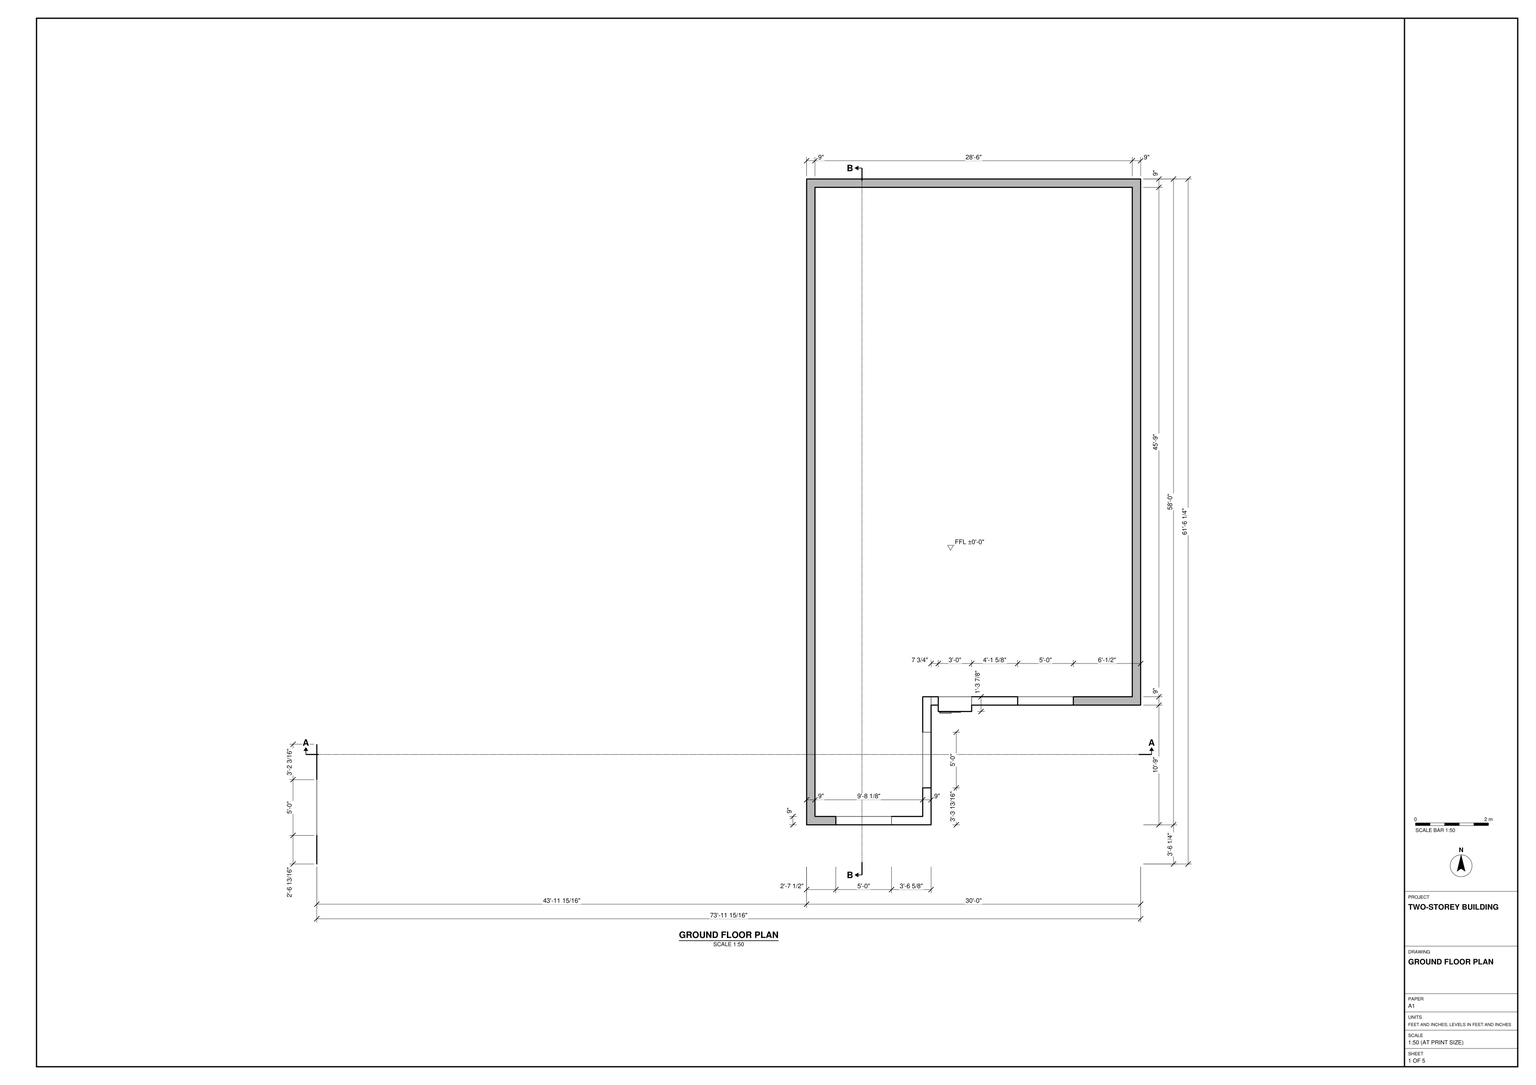
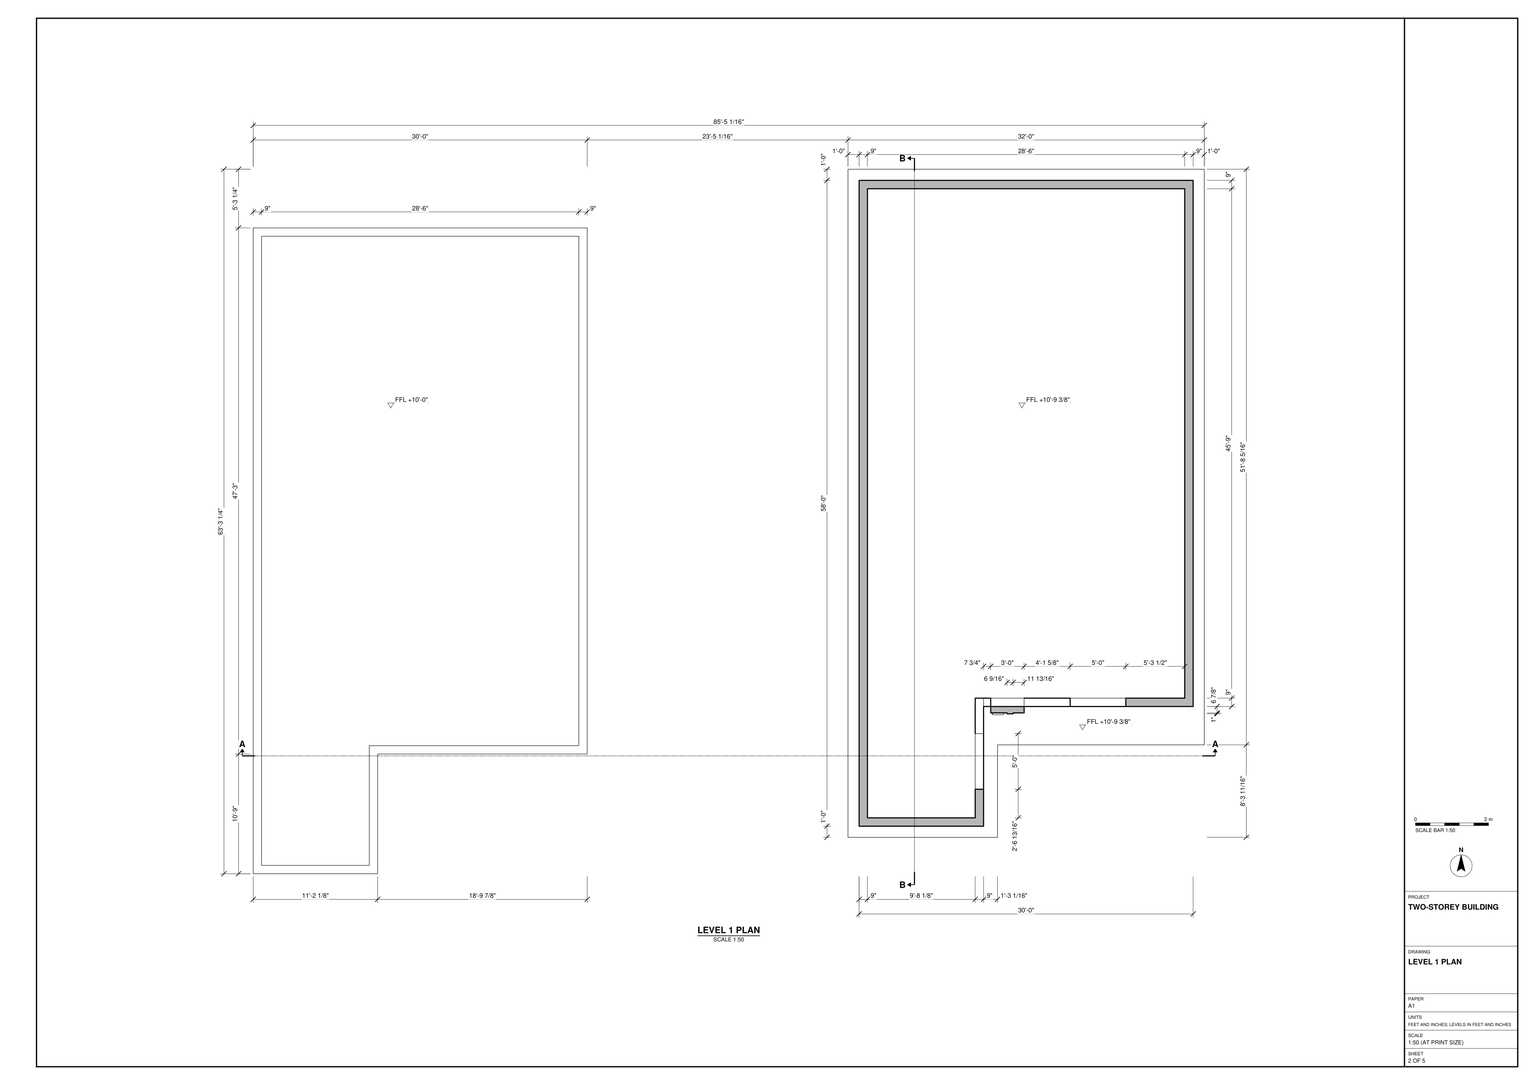
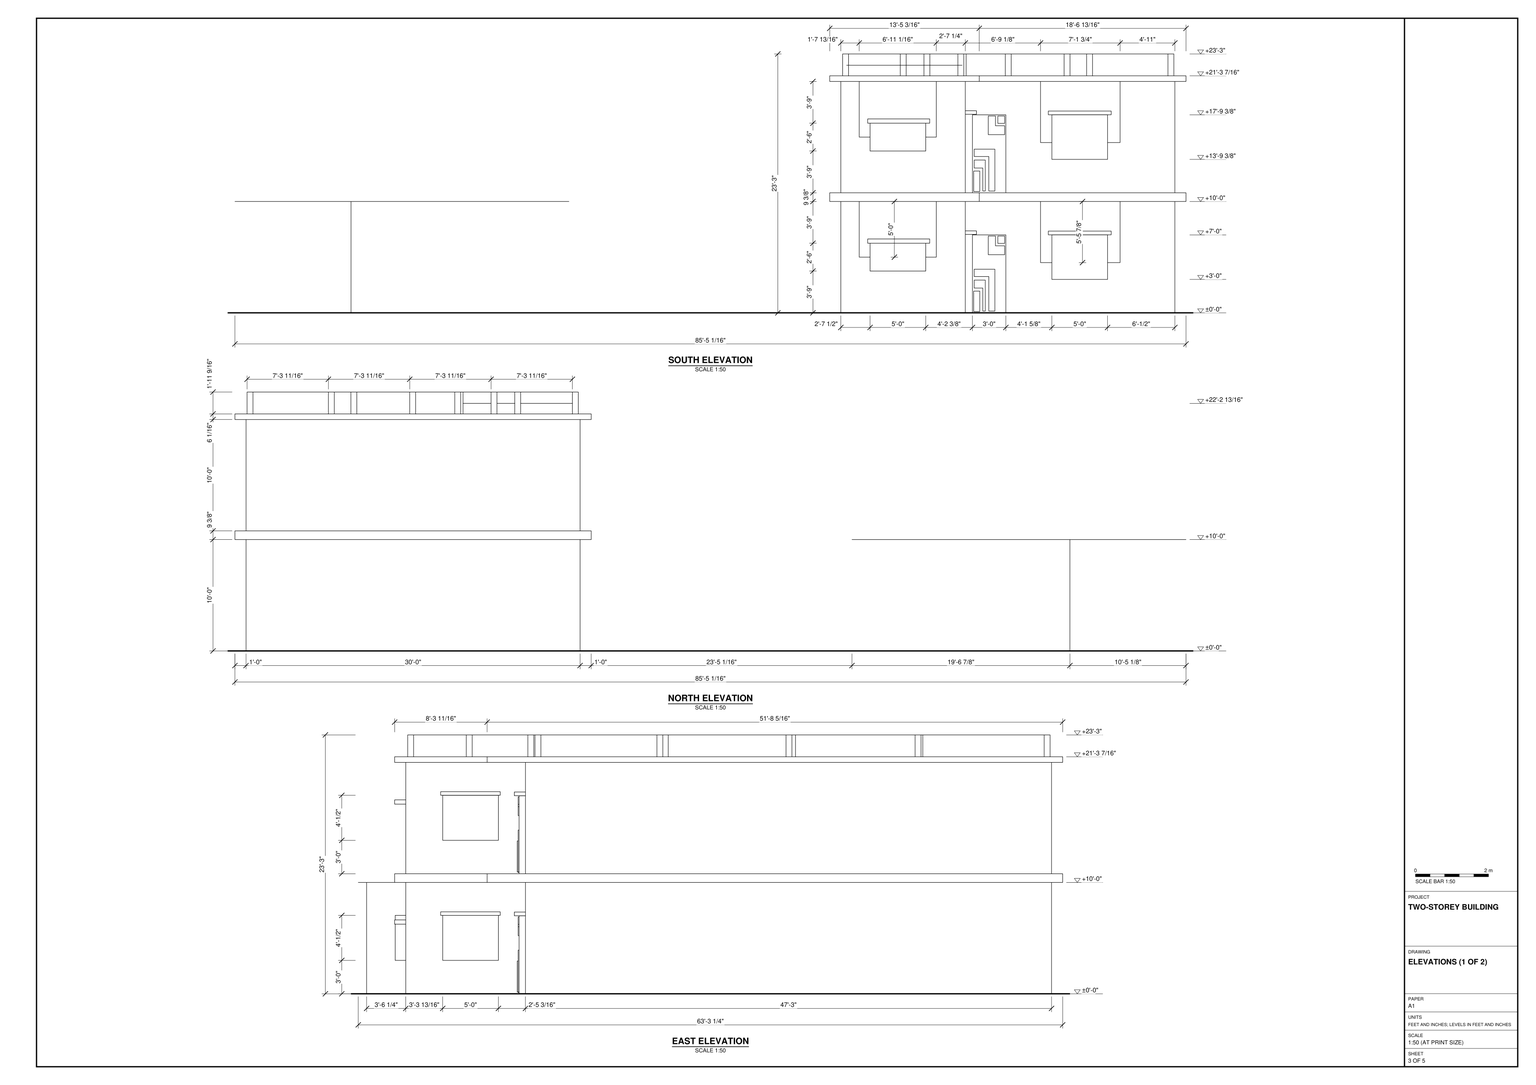
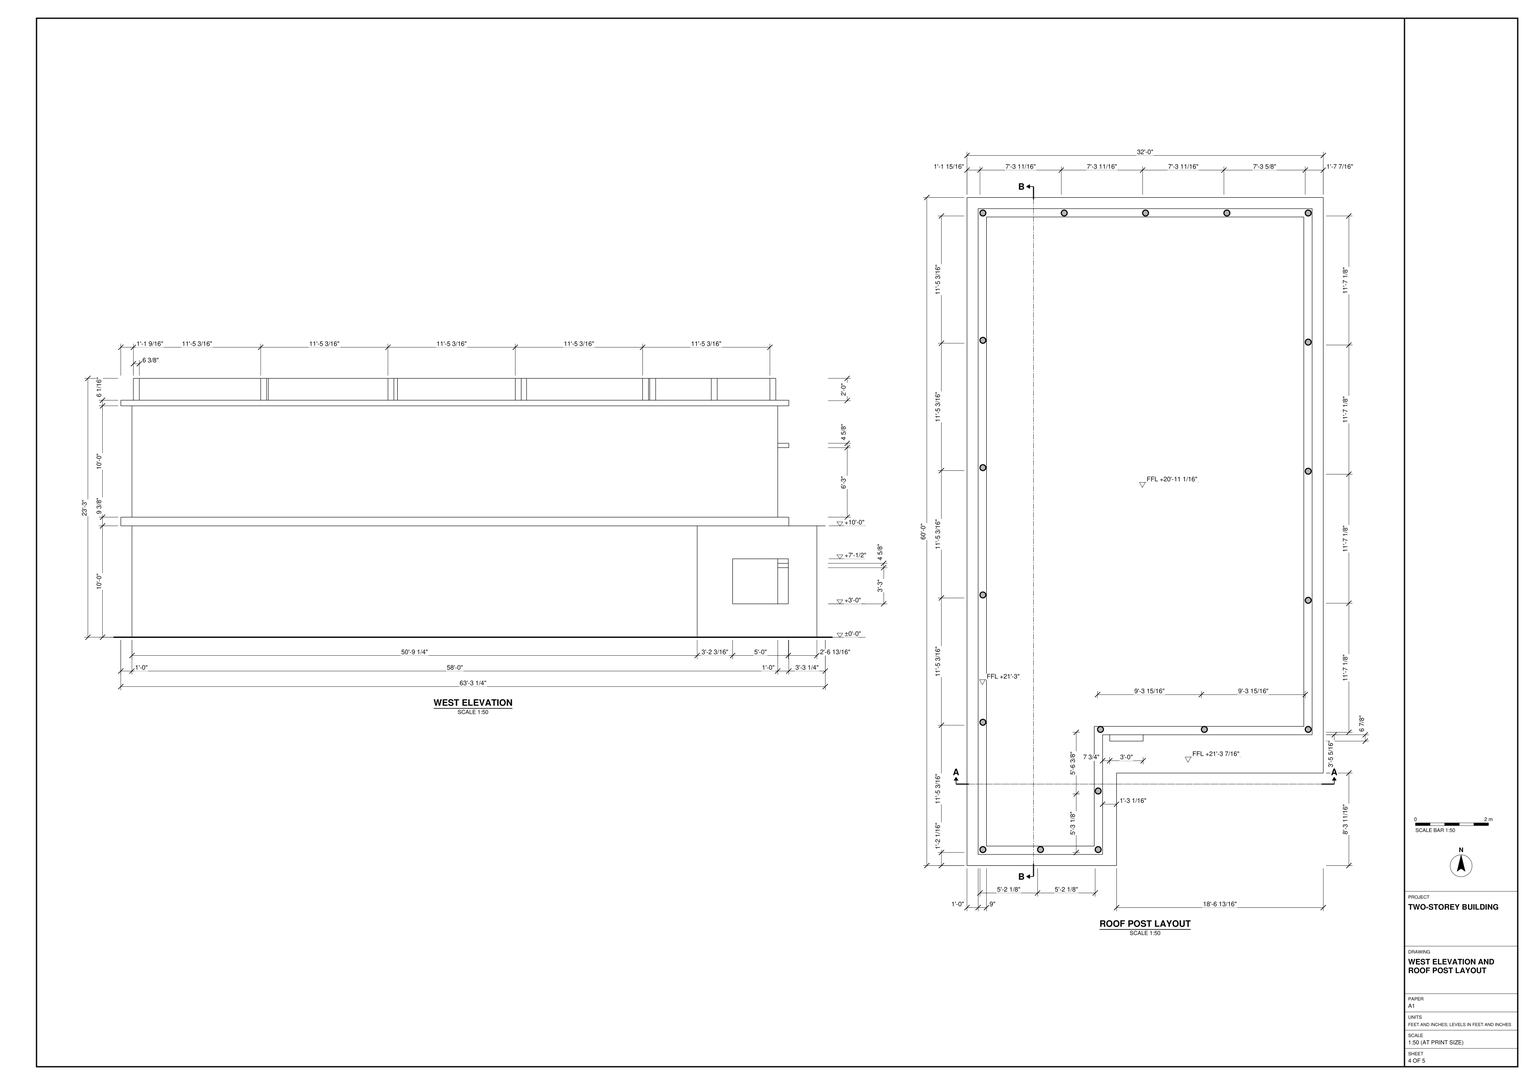
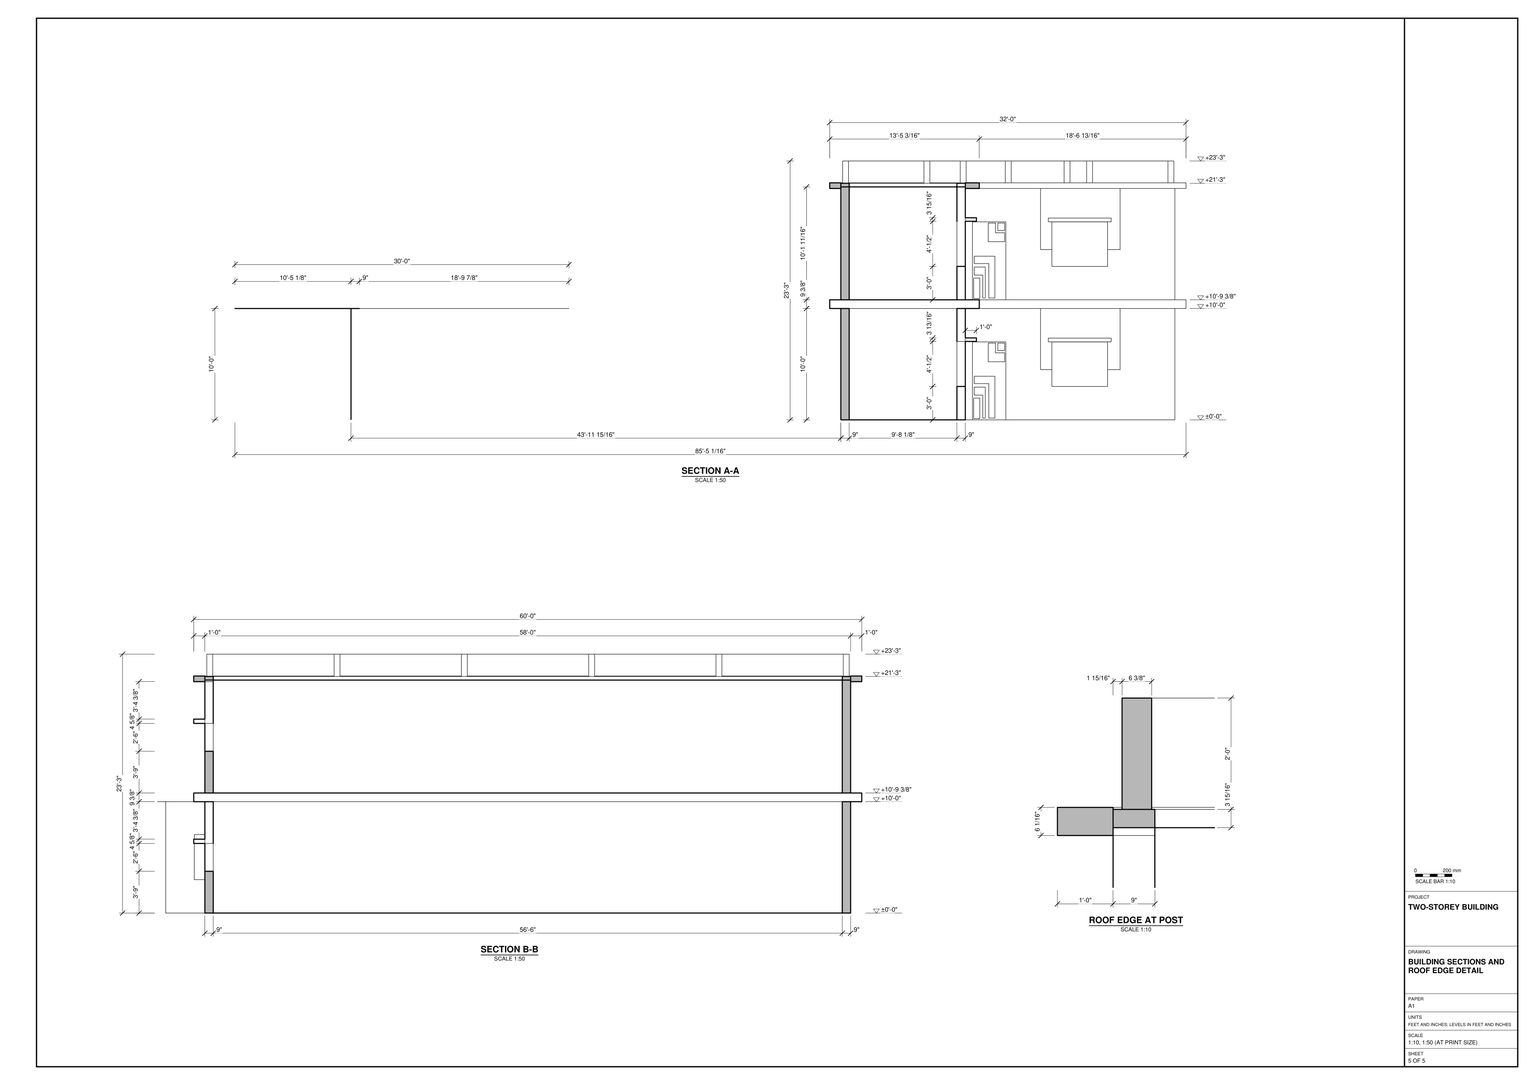
Build the two-storey shell in SketchUp from task_files/diagram_01.pdf. Work in feet and inches. The complete model, including the detached outline, measures 85'-5 1/16" east to west, 63'-3 1/4" north to south and 23'-3" high. Use ±0'-0" for the ground floor and +10'-0" for the upper storey.

Follow the plan for the 9" perimeter walls. The main shell has a broad rectangular portion with a narrow leg projecting south along its west side. Carry this footprint through both storeys. On the south elevation, place the door on the recessed wall, with a window farther along that wall and another on the end of the projecting leg. Use the east elevation to locate the window on the return. Match the openings and their head details on both storeys. Model the projecting intermediate slab, the flat roof slab and the low barrier with uprights around the roof edge. At the upper-floor level, include the separate L-shaped outline west of the shell, preserving its gap and southward offset.

Keep walls, slabs, roof and any furniture or joinery pieces in separate groups or components, and use components for repeated parts. Any decor or loose items shown may use suitable library components. Save one SketchUp model as output_files/two_storey_l_shaped_building_and_its_detached_outline.skp.

# SketchUp Ruby script. Lengths in inches.
U = 1.inch
M = Sketchup.active_model
def pt(a) = Geom::Point3d.new(a.map { |v| v * U })
def face(e, loops, mat)
  f = e.add_face(loops[0].map { |a| pt(a) })
  loops[1..].each { |l| e.add_face(l.map { |a| pt(a) }).erase! }
  f.material = f.back_material = mat if mat
  f
end
# faces: each face lists its corners as indices into pts; further lists are holes
def faces(e, pts, list, mat = nil) = list.each { |f| face(e, (f[0].is_a?(Array) ? f : [f]).map { |l| l.map { |i| pts[i] } }, mat) }
# xy, xz, yz: faces in a plane at the given z, y or x. An outline is a flat list of corners, or four numbers for a rectangle; further outlines are holes
def ring(l) = l.size == 4 ? [[l[0], l[1]], [l[2], l[1]], [l[2], l[3]], [l[0], l[3]]] : l.each_slice(2).to_a
def flat(e, list, mat, &to3) = list.each { |f| face(e, (f[0].is_a?(Array) ? f : [f]).map { |l| ring(l).map { |u, v| to3.(u, v) } }, mat) }
def xy(e, z, list, mat = nil) = flat(e, list, mat) { |x, y| [x, y, z] }
def xz(e, y, list, mat = nil) = flat(e, list, mat) { |x, z| [x, y, z] }
def yz(e, x, list, mat = nil) = flat(e, list, mat) { |y, z| [x, y, z] }
def lines(e, pts, list) = list.each { |a, b| e.add_line(pt(pts[a]), pt(pts[b])) }
# prism: a flat outline (further loops are holes) pulled along v
def prism(e, loops, v, mat = nil)
  f = face(e, loops, mat); d = Geom::Vector3d.new(v.map { |x| x * U })
  f.pushpull(f.normal.samedirection?(d) ? d.length : -d.length)
end
def box(e, o, s, mat = nil) = prism(e, [[o, [o[0] + s[0], o[1], o[2]], [o[0] + s[0], o[1] + s[1], o[2]], [o[0], o[1] + s[1], o[2]]]], [0, 0, s[2]], mat)
def at(x, y, z, deg = 0) = Geom::Transformation.translation(pt([x, y, z])) * Geom::Transformation.rotation(ORIGIN, Z_AXIS, deg.degrees)
def axes(o, x, y, z) = Geom::Transformation.new([*x, 0, *y, 0, *z, 0, *pt(o).to_a, 1])
def part(name) = M.definitions.add(name)
# library, detail: a bought-in or finely detailed component or shape, given as its bounding box
def library(name, o, s) = part(name).tap { |d| box(d.entities, o, s) }
def detail(e, o, s) = box(e.add_group.entities, o, s)
def put(e, d, t, mat = nil) = e.add_instance(d, t).tap { |i| i.material = mat if mat }
def group(e, t, mat = nil) = e.add_group.tap { |g| g.transformation = t; g.material = mat if mat }.entities
root = M.entities
M.materials.add("[0043_SaddleBrown]").color = [139, 69, 19]
M.materials.add("[0045_Goldenrod]").color = [218, 165, 32]
M.materials.add("[Cladding Siding Tan]").color = [162, 126, 95]
M.materials.add("[Color M00]").color = [255, 255, 255]
M.materials.add("[Translucent Glass Blue]").color = [100, 149, 237]
M.materials["[Translucent Glass Blue]"].alpha = 0.5
c1 = part("Cylindrical post")
prism(c1.entities,[[[6.375,3.1875,0],[6.27,2.36,0],[5.95,1.59,0],[5.44,0.93,0],[4.78,0.43,0],[4.01,0.11,0],[3.1875,0,0],[2.36,0.11,0],[1.59,0.43,0],[0.93,0.93,0],[0.43,1.59,0],[0.11,2.36,0],[0,3.1875,0],[0.11,4.01,0],[0.43,4.78,0],[0.93,5.44,0],[1.59,5.95,0],[2.36,6.27,0],[3.1875,6.375,0],[4.01,6.27,0],[4.78,5.95,0],[5.44,5.44,0],[5.95,4.78,0],[6.27,4.01,0]]],[0,0,24])
xy(root,0,[[653.06,51.22,653.06,747.22,1013.06,747.22,1013.06,180.22,940.53,180.22,940.53,189.22,1004.06,189.22,1004.06,738.22,662.06,738.22,662.06,60.22,778.18,60.22,778.18,151.04,787.18,151.04,787.18,51.22],[662.06,60.22,778.18,60.22,778.18,189.22,1004.06,189.22,1004.06,738.22,662.06,738.22],[778.18,151.04,787.18,189.22],[794.9,173.35,830.9,189.22],[787.18,180.22,794.9,189.22],
  [830.9,180.22,940.53,189.22]])
xy(root,1.35,[[796.25,172.35,802.8,173.35]])
xy(root,1.89,[[812.54,172.35,819.08,173.35]])
xy(root,1.91,[[806.07,171.35,808.74,173.35]])
xy(root,23.41,[[796.25,172.35,802.8,173.35]],"[0043_SaddleBrown]")
xy(root,26.68,[[796.82,171.35,806.07,173.35]])
xy(root,35.29,[[796.82,171.35,808.74,173.35]],"[0043_SaddleBrown]")
xy(root,36,[[778.18,91.04,787.18,151.04],[880.53,180.22,940.53,189.22]])
xy(root,39.09,[[796.79,172.35,812.54,173.35]])
xy(root,45,[[684.56,51.22,744.56,60.22]])
xy(root,46.99,[[796.79,172.35,819.08,173.35]],"[0043_SaddleBrown]")
xy(root,62.64,[[811.92,172.35,829.64,173.35]],"[0043_SaddleBrown]")
xy(root,72.24,[[819.7,172.35,829.64,173.35]],"[0043_SaddleBrown]")
xy(root,74.79,[[822.25,172.35,829.62,173.35]],"[0043_SaddleBrown]")
xy(root,74.98,[[682,39.22,684.56,51.22],[744.56,39.22,748.8125,51.22]],"[Color M00]")
xy(root,75,[[684.56,39.22,744.56,51.22]],"[Color M00]")
xy(root,79.61,[[682,39.22,748.8125,51.22]],"[Color M00]")
xy(root,82.71,[[822.25,172.35,829.62,173.35]],"[0043_SaddleBrown]")
xy(root,82.74,[[811.92,172.35,819.7,173.35]],"[0043_SaddleBrown]")
xy(root,84,[[880.53,180.22,940.53,189.22]])
xy(root,84,[[794.9,173.35,830.9,180.22]],"[0043_SaddleBrown]")
xy(root,84.08,[[876.67,168.22,944.42,180.22]],"[Color M00]")
xy(root,84.5,[[787.18,88.8125,799.18,91.04],[787.18,91.04,799.18,151.04],[787.18,151.04,799.18,153]])
xy(root,88.08,[[876.67,168.22,944.42,180.22]],"[Color M00]")
xy(root,88.3125,[[787.18,88.8125,799.18,153]])
xy(root,120,[[[0,0,134.125,0,134.125,129,360,129,360,696,0,696],[9,9,9,687,351,687,351,138,125.125,138,125.125,9]],[9,9,125.125,9,125.125,138,351,138,351,687,9,687],[[641.06,39.22,641.06,759.22,1025.06,759.22,1025.06,138.91,802.24,138.91,802.24,39.22],[653.06,51.22,787.18,51.22,787.18,180.22,1013.06,180.22,1013.06,747.22,653.06,747.22]],[[653.06,51.22,787.18,51.22,787.18,180.22,1013.06,180.22,1013.06,747.22,653.06,747.22],[662.06,60.22,662.06,738.22,1004.06,738.22,1004.06,189.22,778.18,189.22,778.18,60.22]]])
xy(root,129.375,[[[641.06,39.22,802.24,39.22,802.24,138.91,1025.06,138.91,1025.06,759.22,641.06,759.22],[653.06,51.22,653.06,747.22,1013.06,747.22,1013.06,180.22,830.9,180.22,830.9,173.35,794.9,173.35,794.9,180.22,787.18,180.22,787.18,51.22]],[653.06,51.22,653.06,747.22,1013.06,747.22,1013.06,180.22,940.53,180.22,940.53,189.22,1004.06,189.22,1004.06,738.22,662.06,738.22,662.06,60.22,744.56,60.22,744.56,51.22],[744.56,51.22,787.18,60.15],[744.56,60.15,744.56,60.22,778.18,60.22,778.18,151.04,787.18,151.04,787.18,60.15],[662.06,60.22,778.18,60.22,778.18,189.22,1004.06,189.22,1004.06,738.22,662.06,738.22],
  [778.18,151.04,787.18,189.22],[794.9,173.35,830.9,180.22],[787.18,180.22,794.9,189.22],[794.9,180.22,830.9,189.22],[830.9,180.22,940.53,189.22]])
xy(root,130.72,[[796.25,172.35,802.8,173.35]])
xy(root,131.26,[[812.54,172.35,819.08,173.35]])
xy(root,131.29,[[806.07,171.35,808.74,173.35]])
xy(root,152.79,[[796.25,172.35,802.8,173.35]],"[0043_SaddleBrown]")
xy(root,156.05,[[796.82,171.35,806.07,173.35]])
xy(root,164.67,[[796.82,171.35,808.74,173.35]],"[0043_SaddleBrown]")
xy(root,165.375,[[778.18,91.04,787.18,151.04],[880.53,180.22,940.53,189.22]])
xy(root,168.47,[[796.79,172.35,812.54,173.35]])
xy(root,174.375,[[684.56,51.22,744.56,60.22]])
xy(root,176.37,[[796.79,172.35,819.08,173.35]],"[0043_SaddleBrown]")
xy(root,192.01,[[811.92,172.35,829.64,173.35]],"[0043_SaddleBrown]")
xy(root,201.61,[[819.7,172.35,829.64,173.35]],"[0043_SaddleBrown]")
xy(root,204.16,[[822.25,172.35,829.62,173.35]],"[0043_SaddleBrown]")
xy(root,204.36,[[682,39.22,684.56,51.22],[744.56,39.22,748.8125,51.22]],"[Color M00]")
xy(root,204.375,[[684.56,39.22,744.56,51.22]],"[Color M00]")
xy(root,208.98,[[682,39.22,748.8125,51.22]],"[Color M00]")
xy(root,212.09,[[822.25,172.35,829.62,173.35]],"[0043_SaddleBrown]")
xy(root,212.11,[[811.92,172.35,819.7,173.35]],"[0043_SaddleBrown]")
xy(root,213.375,[[880.53,180.22,940.53,189.22]])
xy(root,213.375,[[794.9,173.35,830.9,180.22]],"[0043_SaddleBrown]")
xy(root,213.45,[[876.67,168.22,944.42,180.22]],"[Color M00]")
xy(root,213.98,[[787.18,88.8125,799.18,153]])
xy(root,217.45,[[876.67,168.22,944.42,180.22]],"[Color M00]")
xy(root,217.8,[[787.18,88.8125,799.18,153]])
xy(root,249.375,[[[641.06,39.22,641.06,759.22,1025.06,759.22,1025.06,138.91,802.24,138.91,802.24,39.22],[653.06,51.22,787.18,51.22,787.18,180.22,794.9,180.22,794.9,173.35,830.9,173.35,830.9,180.22,1013.06,180.22,1013.06,747.22,653.06,747.22]]])
xy(root,251.0625,[[653.06,51.22,787.18,51.22,787.18,180.22,1013.06,180.22,1013.06,747.22,653.06,747.22]])
xy(root,255,[[[653.06,51.22,787.18,51.22,787.18,180.22,1013.06,180.22,1013.06,747.22,653.06,747.22],[662.06,60.22,662.06,738.22,1004.06,738.22,1004.06,189.22,778.18,189.22,778.18,60.22]]])
xy(root,255.4375,[[[641.06,39.22,802.24,39.22,802.24,138.91,1025.06,138.91,1025.06,759.22,641.06,759.22],[653.06,51.22,653.06,747.22,1013.06,747.22,1013.06,180.22,830.9,180.22,830.9,173.35,794.9,173.35,794.9,180.22,787.18,180.22,787.18,51.22]],[794.9,173.35,830.9,180.22]])
xz(root,39.22,[[641.06,120,802.24,129.375],[641.06,249.375,802.24,255.4375]])
xz(root,39.22,[[682,74.98,684.56,74.98,684.56,75,744.56,75,744.56,74.98,748.8125,74.98,748.8125,79.61,682,79.61],[682,204.36,684.56,204.36,684.56,204.375,744.56,204.375,744.56,204.36,748.8125,204.36,748.8125,208.98,682,208.98]],"[Color M00]")
xz(root,51.22,[[653.06,0,787.18,0,787.18,120,755.93,120,755.93,60,744.56,60,744.56,45,684.56,45,684.56,60,672.87,60,672.87,120,653.06,120],[653.06,129.375,787.18,129.375,787.18,249.375,755.93,249.375,755.93,189.375,744.56,189.375,744.56,174.375,684.56,174.375,684.56,189.375,672.87,189.375,672.87,249.375,653.06,249.375],[653.06,249.375,672.87,251.0625],[672.87,249.375,744.56,251.0625],[744.56,249.375,755.93,251.0625],
  [755.93,249.375,787.18,251.0625],[653.06,251.0625,672.87,255],[672.87,251.0625,744.56,255],[744.56,251.0625,755.93,255],[755.93,251.0625,787.18,255],
  [653.06,255,672.87,255.4375],[672.87,255,744.56,255.4375],[744.56,255,755.93,255.4375],[755.93,255,787.18,255.4375]])
xz(root,51.22,[[672.87,60,684.56,60,684.56,74.98,682,74.98,682,79.61,748.8125,79.61,748.8125,74.98,744.56,74.98,744.56,60,755.93,60,755.93,120,672.87,120],[672.87,189.375,684.56,189.375,684.56,204.36,682,204.36,682,208.98,748.8125,208.98,748.8125,204.36,744.56,204.36,744.56,189.375,755.93,189.375,755.93,249.375,672.87,249.375]],"[Cladding Siding Tan]")
xz(root,51.22,[[684.56,45,744.56,74.98],[684.56,74.98,744.56,75],[684.56,174.375,744.56,204.36],[684.56,204.36,744.56,204.375]],"[Translucent Glass Blue]")
xz(root,60.22,[[[662.06,0,778.18,120],[684.56,45,744.56,75]],[[662.06,129.375,778.18,255],[684.56,174.375,744.56,204.375]]])
xz(root,88.8125,[[787.18,84.5,799.18,88.3125],[787.18,213.98,799.18,217.8]])
xz(root,91.04,[[778.18,36,787.18,84.5],[778.18,165.375,787.18,213.875]])
xz(root,138.91,[[802.24,120,1025.06,129.375],[802.24,249.375,1025.06,255.4375]])
xz(root,153,[[787.18,84.5,799.18,88.3125],[787.18,213.98,799.18,217.8]])
xz(root,168.22,[[876.67,84.08,944.42,88.08],[876.67,213.45,944.42,217.45]],"[Color M00]")
xz(root,171.35,[[806.07,1.91,808.74,1.91,808.74,35.29,796.82,35.29,796.82,26.68,806.07,26.68],[806.07,131.29,808.74,131.29,808.74,164.67,796.82,164.67,796.82,156.05,806.07,156.05]],"[0043_SaddleBrown]")
xz(root,172.35,[[796.25,1.35,802.8,23.41],[812.54,1.89,819.08,1.89,819.08,46.99,796.79,46.99,796.79,39.09,812.54,39.09],[811.92,62.64,829.64,62.64,829.64,72.24,819.7,72.24,819.7,82.74,811.92,82.74],[822.25,74.79,829.62,82.71],[796.25,130.72,802.8,152.79],
  [812.54,131.26,819.08,131.26,819.08,176.37,796.79,176.37,796.79,168.47,812.54,168.47],[811.92,192.01,829.64,192.01,829.64,201.61,819.7,201.61,819.7,212.11,811.92,212.11],[822.25,204.16,829.62,212.09]],"[0043_SaddleBrown]")
xz(root,173.35,[[794.9,249.375,830.9,255.4375]])
xz(root,173.35,[[[794.9,0,830.9,84],[812.54,1.89,812.54,39.09,796.79,39.09,796.79,46.99,819.08,46.99,819.08,1.89],[811.92,62.64,811.92,82.74,819.7,82.74,819.7,72.24,829.64,72.24,829.64,62.64],[806.07,1.91,806.07,26.68,796.82,26.68,796.82,35.29,808.74,35.29,808.74,1.91],[796.25,1.35,802.8,23.41],[822.25,74.79,829.62,82.71]],[[794.9,129.375,830.9,213.375],[812.54,131.26,812.54,168.47,796.79,168.47,796.79,176.37,819.08,176.37,819.08,131.26],[811.92,192.01,811.92,212.11,819.7,212.11,819.7,201.61,829.64,201.61,829.64,192.01],[806.07,131.29,806.07,156.05,796.82,156.05,796.82,164.67,808.74,164.67,808.74,131.29],[796.25,130.72,802.8,152.79],[822.25,204.16,829.62,212.09]]],"[0045_Goldenrod]")
xz(root,180.22,[[787.18,0,794.9,0,794.9,84,830.9,84,830.9,0,1013.06,0,1013.06,120,954.03,120,954.03,54.125,940.53,54.125,940.53,36,880.53,36,880.53,54.125,868.28,54.125,868.28,120,787.18,120],[787.18,129.375,794.9,129.375,794.9,213.375,830.9,213.375,830.9,129.375,1013.06,129.375,1013.06,249.375,954.03,249.375,954.03,183.5,940.53,183.5,940.53,165.375,880.53,165.375,880.53,183.5,868.28,183.5,868.28,249.375,830.9,249.375,830.9,251.0625,794.9,251.0625,794.9,249.375,787.18,249.375],[794.9,129.375,830.9,213.375],[787.18,249.375,794.9,251.0625],[830.9,249.375,868.28,251.0625],
  [868.28,249.375,940.53,251.0625],[940.53,249.375,954.03,251.0625],[954.03,249.375,1013.06,251.0625],[787.18,251.0625,794.9,255],[794.9,251.0625,830.9,255],
  [830.9,251.0625,868.28,255],[868.28,251.0625,940.53,255],[940.53,251.0625,954.03,255],[954.03,251.0625,1013.06,255],[787.18,255,794.9,255.4375],
  [794.9,255,830.9,255.4375],[830.9,255,868.28,255.4375],[868.28,255,940.53,255.4375],[940.53,255,954.03,255.4375],[954.03,255,1013.06,255.4375]])
xz(root,180.22,[[[868.28,54.125,880.53,54.125,880.53,84,940.53,84,940.53,54.125,954.03,54.125,954.03,120,868.28,120],[876.67,84.08,944.42,88.08]],[[868.28,183.5,880.53,183.5,880.53,213.375,940.53,213.375,940.53,183.5,954.03,183.5,954.03,249.375,868.28,249.375],[876.67,213.45,944.42,217.45]]],"[Cladding Siding Tan]")
xz(root,180.22,[[880.53,36,940.53,84],[880.53,165.375,940.53,213.375]],"[Translucent Glass Blue]")
xz(root,189.22,[[[778.18,0,778.18,120,1004.06,120,1004.06,0,830.9,0,830.9,84,794.9,84,794.9,0],[880.53,36,940.53,84]],[[778.18,129.375,778.18,255,1004.06,255,1004.06,129.375,830.9,129.375,830.9,213.375,794.9,213.375,794.9,129.375],[880.53,165.375,940.53,213.375]]])
xz(root,738.22,[[662.06,0,1004.06,120],[662.06,129.375,1004.06,255]])
xz(root,747.22,[[653.06,0,1013.06,120],[653.06,129.375,1013.06,249.375],[653.06,249.375,1013.06,251.0625],[653.06,251.0625,1013.06,255],[653.06,255,1013.06,255.4375]])
xz(root,759.22,[[641.06,120,1025.06,129.375],[641.06,249.375,1025.06,255.4375]])
yz(root,125.125,[[[9,0,138,120],[39.82,36,99.82,84.5]]])
yz(root,641.06,[[39.22,120,759.22,129.375],[39.22,249.375,759.22,255.4375]])
yz(root,653.06,[[51.22,0,747.22,120],[51.22,129.375,747.22,249.375],[51.22,249.375,747.22,251.0625],[51.22,251.0625,747.22,255],[51.22,255,747.22,255.4375]])
yz(root,662.06,[[60.22,0,738.22,120],[60.22,129.375,738.22,255]])
yz(root,682,[[39.22,74.98,51.22,79.61],[39.22,204.36,51.22,208.98]],"[Color M00]")
yz(root,684.56,[[51.22,45,60.22,75],[51.22,174.375,60.22,204.375]])
yz(root,684.56,[[39.22,74.98,51.22,75],[39.22,204.36,51.22,204.375]],"[Cladding Siding Tan]")
yz(root,744.56,[[39.22,74.98,51.22,75],[39.22,204.36,51.22,204.375]],"[Cladding Siding Tan]")
yz(root,748.8125,[[39.22,74.98,51.22,79.61],[39.22,204.36,51.22,208.98]],"[Color M00]")
yz(root,778.18,[[[60.22,0,189.22,120],[91.04,36,151.04,84.5]],[[60.22,129.375,189.22,255],[91.04,165.375,151.04,213.875]]])
yz(root,787.18,[[[51.22,0,180.22,120],[91.04,36,91.04,84.5,88.8125,84.5,88.8125,88.3125,153,88.3125,153,84.5,151.04,84.5,151.04,36]],[[51.22,129.375,180.22,249.375],[91.04,165.375,151.04,213.875],[88.8125,213.98,153,217.8]],[51.22,249.375,60.15,251.0625],[60.15,249.375,151.04,251.0625],[151.04,249.375,180.22,251.0625],
  [51.22,251.0625,60.15,255],[60.15,251.0625,151.04,255],[151.04,251.0625,180.22,255],[51.22,255,60.15,255.4375],[60.15,255,151.04,255.4375],
  [151.04,255,180.22,255.4375]])
yz(root,787.18,[[91.04,36,151.04,84.5],[91.04,165.375,151.04,213.875]],"[Translucent Glass Blue]")
yz(root,794.9,[[180.22,0,189.22,84],[180.22,129.375,189.22,213.375],[173.35,249.375,180.22,255.4375]])
yz(root,794.9,[[173.35,0,180.22,84],[173.35,129.375,180.22,213.375]],"[0043_SaddleBrown]")
yz(root,796.25,[[172.35,1.35,173.35,23.41],[172.35,130.72,173.35,152.79]],"[0043_SaddleBrown]")
yz(root,796.79,[[172.35,39.09,173.35,46.99],[172.35,168.47,173.35,176.37]],"[0043_SaddleBrown]")
yz(root,796.82,[[171.35,26.68,173.35,35.29],[171.35,156.05,173.35,164.67]],"[0043_SaddleBrown]")
yz(root,799.18,[[88.8125,84.5,153,88.3125],[88.8125,213.98,153,217.8]])
yz(root,802.24,[[39.22,120,138.91,129.375],[39.22,249.375,138.91,255.4375]])
yz(root,802.8,[[172.35,1.35,173.35,23.41],[172.35,130.72,173.35,152.79]],"[0043_SaddleBrown]")
yz(root,806.07,[[171.35,1.91,173.35,26.68],[171.35,131.29,173.35,156.05]],"[0043_SaddleBrown]")
yz(root,808.74,[[171.35,1.91,173.35,35.29],[171.35,131.29,173.35,164.67]],"[0043_SaddleBrown]")
yz(root,811.92,[[172.35,62.64,173.35,82.74],[172.35,192.01,173.35,212.11]],"[0043_SaddleBrown]")
yz(root,812.54,[[172.35,1.89,173.35,39.09],[172.35,131.26,173.35,168.47]],"[0043_SaddleBrown]")
yz(root,819.08,[[172.35,1.89,173.35,46.99],[172.35,131.26,173.35,176.37]],"[0043_SaddleBrown]")
yz(root,819.7,[[172.35,72.24,173.35,82.74],[172.35,201.61,173.35,212.11]],"[0043_SaddleBrown]")
yz(root,822.25,[[172.35,74.79,173.35,82.71],[172.35,204.16,173.35,212.09]],"[0043_SaddleBrown]")
yz(root,829.62,[[172.35,74.79,173.35,82.71],[172.35,204.16,173.35,212.09]],"[0043_SaddleBrown]")
yz(root,829.64,[[172.35,62.64,173.35,72.24],[172.35,192.01,173.35,201.61]],"[0043_SaddleBrown]")
yz(root,830.9,[[173.35,249.375,180.22,255.4375]])
yz(root,830.9,[[173.35,0,180.22,84],[173.35,129.375,180.22,213.375]],"[0043_SaddleBrown]")
yz(root,876.67,[[168.22,84.08,180.22,88.08],[168.22,213.45,180.22,217.45]],"[Color M00]")
yz(root,880.53,[[180.22,36,189.22,84],[180.22,165.375,189.22,213.375]])
yz(root,940.53,[[180.22,36,189.22,84],[180.22,165.375,189.22,213.375]])
yz(root,944.42,[[168.22,84.08,180.22,88.08],[168.22,213.45,180.22,217.45]],"[Color M00]")
yz(root,1004.06,[[189.22,0,738.22,120],[189.22,129.375,738.22,255]])
yz(root,1013.06,[[180.22,0,747.22,120],[180.22,129.375,747.22,249.375],[180.22,249.375,747.22,251.0625],[180.22,251.0625,747.22,255],[180.22,255,747.22,255.4375]])
yz(root,1025.06,[[138.91,120,759.22,129.375],[138.91,249.375,759.22,255.4375]])
p = [[854.9,180.22,84],[854.9,189.22,84],[787.18,164.29,84.5],[778.18,164.29,84.5],[744.56,60.15,0],[744.56,60.22,0],
  [746.12,51.22,75],[746.12,60.22,75],[787.18,51.22,129.375],[787.18,51.22,120],[659.24,53.5,266.79],[718.98,53.5,266.79],
  [783.78,53.5,266.79],[661.25,55.66,279],[717.21,55.66,279],[781.57,53.4,279],[783.99,116.85,279],[783.99,185.1,279],
  [902.98,185.1,279],[1011.88,185.1,279],[1011.88,322.85,279],[1011.88,743.31,279],[661.25,743.31,279],[661.25,58.1,279]]
lines(root,p,[[0,1],[2,3],[4,5],[6,7],[8,9],[10,11],[11,12],[13,14],[14,15],[15,16],[16,17],[17,18],
  [18,19],[19,20],[20,21],[21,22],[22,23]])
put(root,c1,at(654.99,53.29,255))
put(root,c1,at(717.1,53.29,255))
put(root,c1,at(779.21,53.29,255))
put(root,c1,at(654.99,190.49,255))
put(root,c1,at(654.99,327.69,255))
put(root,c1,at(654.99,464.89,255))
put(root,c1,at(654.99,602.09,255))
put(root,c1,at(654.99,739.29,255))
put(root,c1,at(742.64,739.29,255))
put(root,c1,at(830.3,739.29,255))
put(root,c1,at(917.96,739.29,255))
put(root,c1,at(1005.61,739.29,255))
put(root,c1,at(1005.61,600.17,255))
put(root,c1,at(1005.61,461.04,255))
put(root,c1,at(1005.61,321.92,255))
put(root,c1,at(1005.61,182.79,255))
put(root,c1,at(893.68,182.79,255))
put(root,c1,at(781.74,182.79,255))
put(root,c1,at(779.21,116.42,255))
